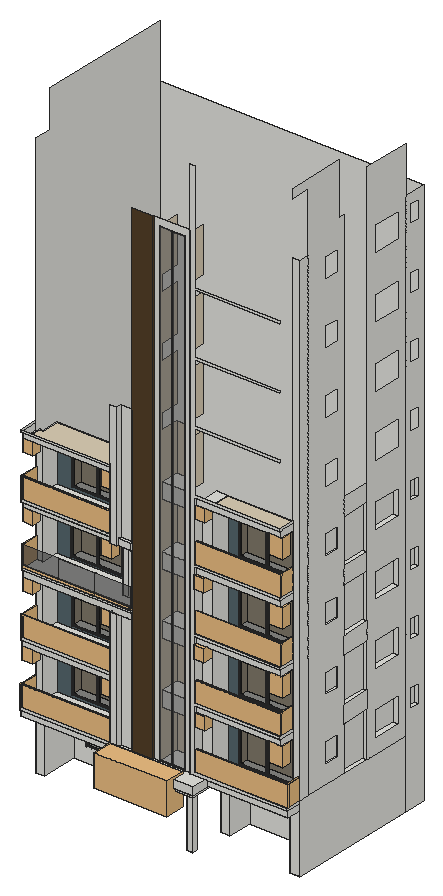
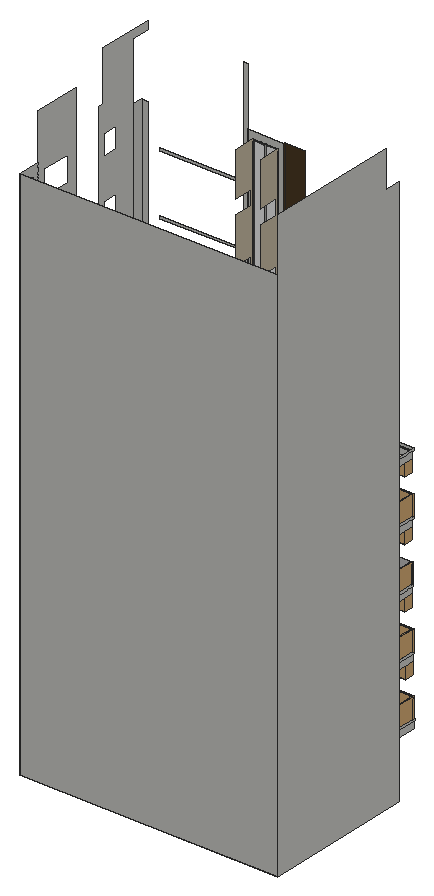
# SketchUp Ruby script. Lengths in inches.
U = 1.inch
M = Sketchup.active_model
def pt(a) = Geom::Point3d.new(a.map { |v| v * U })
def face(e, loops, mat)
  f = e.add_face(loops[0].map { |a| pt(a) })
  loops[1..].each { |l| e.add_face(l.map { |a| pt(a) }).erase! }
  f.material = f.back_material = mat if mat
  f
end
# faces: each face lists its corners as indices into pts; further lists are holes
def faces(e, pts, list, mat = nil) = list.each { |f| face(e, (f[0].is_a?(Array) ? f : [f]).map { |l| l.map { |i| pts[i] } }, mat) }
# xy, xz, yz: faces in a plane at the given z, y or x. An outline is a flat list of corners, or four numbers for a rectangle; further outlines are holes
def ring(l) = l.size == 4 ? [[l[0], l[1]], [l[2], l[1]], [l[2], l[3]], [l[0], l[3]]] : l.each_slice(2).to_a
def flat(e, list, mat, &to3) = list.each { |f| face(e, (f[0].is_a?(Array) ? f : [f]).map { |l| ring(l).map { |u, v| to3.(u, v) } }, mat) }
def xy(e, z, list, mat = nil) = flat(e, list, mat) { |x, y| [x, y, z] }
def xz(e, y, list, mat = nil) = flat(e, list, mat) { |x, z| [x, y, z] }
def yz(e, x, list, mat = nil) = flat(e, list, mat) { |y, z| [x, y, z] }
def lines(e, pts, list) = list.each { |a, b| e.add_line(pt(pts[a]), pt(pts[b])) }
# prism: a flat outline (further loops are holes) pulled along v
def prism(e, loops, v, mat = nil)
  f = face(e, loops, mat); d = Geom::Vector3d.new(v.map { |x| x * U })
  f.pushpull(f.normal.samedirection?(d) ? d.length : -d.length)
end
def box(e, o, s, mat = nil) = prism(e, [[o, [o[0] + s[0], o[1], o[2]], [o[0] + s[0], o[1] + s[1], o[2]], [o[0], o[1] + s[1], o[2]]]], [0, 0, s[2]], mat)
def at(x, y, z, deg = 0) = Geom::Transformation.translation(pt([x, y, z])) * Geom::Transformation.rotation(ORIGIN, Z_AXIS, deg.degrees)
def axes(o, x, y, z) = Geom::Transformation.new([*x, 0, *y, 0, *z, 0, *pt(o).to_a, 1])
def part(name) = M.definitions.add(name)
# library, detail: a bought-in or finely detailed component or shape, given as its bounding box
def library(name, o, s) = part(name).tap { |d| box(d.entities, o, s) }
def detail(e, o, s) = box(e.add_group.entities, o, s)
def put(e, d, t, mat = nil) = e.add_instance(d, t).tap { |i| i.material = mat if mat }
def group(e, t, mat = nil) = e.add_group.tap { |g| g.transformation = t; g.material = mat if mat }.entities
root = M.entities
M.materials.add("Glass_Tinted_Gray").color = [0, 0, 0]
M.materials["Glass_Tinted_Gray"].alpha = 0.125
M.materials.add("Wall Paint Bumpy 01 Blue 100cm").color = [86, 103, 109]
M.materials.add("Wood Planks Pecan 33-81 150cm").color = [83, 63, 40]
M.materials.add("[0135_DarkGray]").color = [81, 81, 81]
M.materials.add("[Mirror 02]").color = [96, 96, 96]
M.materials["[Mirror 02]"].alpha = 0.27
M.materials.add("[Terrazzo Light Blue]").color = [196, 214, 227]
M.materials.add("[Translucent_Glass_Blue]").color = [63, 63, 63]
M.materials["[Translucent_Glass_Blue]"].alpha = 0.35
M.materials.add("metal railing").color = [165, 165, 165]
M.materials.add("plastic2").color = [86, 86, 86]
M.materials.add("warmk").color = [218, 205, 180]
c1 = part("PENTEK_RP Fineline 50S_Sliding_DoorCase_E1")
box(c1.entities,[0,0,0],[1.51,3.66,99.27],"[0135_DarkGray]")
c2 = part("PENTEK_RP Fineline 50S_SlidingDooe_Case_E2")
box(c2.entities,[0,0,0],[96.25,3.66,1.51],"[0135_DarkGray]")
c3 = part("pentek_RP Fineline 50S_SlidingDoor_Case")
put(c3.entities,c1,at(97.76,0,0))
put(c3.entities,c2,at(1.51,0,0))
put(c3.entities,c1,at(0,0,0))
put(c3.entities,c2,at(1.51,0,97.76))
c4 = part("PENTEK_RP Fineline 50S_SlidingDoor_GlazingBead_2")
box(c4.entities,[0,0,0],[0.56,0.59,94.39],"[0135_DarkGray]")
c5 = part("PENTEK_RP Fineline 50S_SlidingDoor_GlazingBead")
box(c5.entities,[0,0,0],[45.47,0.59,0.56],"[0135_DarkGray]")
c6 = part("PENTEK_RP Fineline 50S_SlidingDoor_Glass")
box(c6.entities,[0,0,0],[46.58,0.16,94.39],"Glass_Tinted_Gray")
c7 = part("PENTEK_RP Fineline 50S_SlidingDoor_Leaf_E1")
xy(c7.entities,0,[[0,0,0.93,1.97],[0.93,1.57,1.49,1.97]],"[0135_DarkGray]")
xy(c7.entities,96.25,[[0,0,0.93,0,0.93,1.57,1.49,1.57,1.49,1.97,0,1.97]],"[0135_DarkGray]")
xz(c7.entities,0,[[0,0,0.93,96.25]],"[0135_DarkGray]")
xz(c7.entities,1.57,[[0.93,0,1.49,95.32],[0.93,95.32,1.49,96.25]],"[0135_DarkGray]")
xz(c7.entities,1.97,[[0,0,1.49,96.25]],"[0135_DarkGray]")
yz(c7.entities,0,[[0,0,1.97,96.25]],"[0135_DarkGray]")
yz(c7.entities,0.93,[[0,0,1.57,0.93],[0,0.93,1.57,95.32],[0,95.32,1.57,96.25]],"[0135_DarkGray]")
yz(c7.entities,1.49,[[1.57,0,1.97,95.32],[1.57,95.32,1.97,96.25]],"[0135_DarkGray]")
c8 = part("PENTEK_RP Fineline 50S_SlidingDoor_Leaf_E2")
xy(c8.entities,0,[[0,0,0,1.57,0.56,1.57,0.56,1.97,46.02,1.97,46.02,1.57,46.58,1.57,46.58,0]],"[0135_DarkGray]")
xy(c8.entities,0.93,[[0,0,46.58,1.57]],"[0135_DarkGray]")
xy(c8.entities,1.49,[[0.56,1.57,46.02,1.97]],"[0135_DarkGray]")
xz(c8.entities,0,[[0,0,46.58,0.93]],"[0135_DarkGray]")
xz(c8.entities,1.57,[[0,0,0.56,0.93],[46.02,0,46.58,0.93],[0.56,0.93,46.02,1.49]],"[0135_DarkGray]")
xz(c8.entities,1.97,[[0.56,0,46.02,1.49]],"[0135_DarkGray]")
yz(c8.entities,0,[[0,0,1.57,0.93]],"[0135_DarkGray]")
yz(c8.entities,0.56,[[1.57,0,1.97,0.93],[1.57,0.93,1.97,1.49]],"[0135_DarkGray]")
yz(c8.entities,46.02,[[1.57,0,1.97,0.93],[1.57,0.93,1.97,1.49]],"[0135_DarkGray]")
yz(c8.entities,46.58,[[0,0,1.57,0.93]],"[0135_DarkGray]")
c9 = part("PENTEK_RP Fineline S_SlidingDoor_Leaf1")
put(c9.entities,c4,at(0.93,0,0.93))
put(c9.entities,c4,at(46.96,0,0.93))
put(c9.entities,c5,at(1.49,0,0.93))
put(c9.entities,c6,at(1.49,0.59,0.93),"[Terrazzo Light Blue]")
put(c9.entities,c7,at(0,0,0))
put(c9.entities,c7,axes([48.44,0,0],[-1,0,0],[0,1,0],[0,0,1]))
put(c9.entities,c8,axes([0.93,0,96.25],[1,0,0],[0,1,0],[0,0,-1]))
put(c9.entities,c5,at(1.49,0,94.77))
put(c9.entities,c6,at(1.49,1.42,0.93))
put(c9.entities,c8,at(0.93,0,0))
c10 = part("PENTEK_RP Fineline 50S_SlidingDoor_Leaf2")
put(c10.entities,c6,at(1.49,1.42,0.93))
put(c10.entities,c5,at(1.49,0,94.77))
put(c10.entities,c4,at(46.96,0,0.93))
put(c10.entities,c6,at(1.49,0.59,0.93),"[Mirror 02]")
put(c10.entities,c4,at(0.93,0,0.93))
put(c10.entities,c7,at(0,0,0))
put(c10.entities,c7,axes([48.44,0,0],[-1,0,0],[0,1,0],[0,0,1]))
put(c10.entities,c5,at(1.49,0,0.93))
put(c10.entities,c8,axes([0.93,0,96.25],[1,0,0],[0,1,0],[0,0,-1]))
put(c10.entities,c8,at(0.93,0,0))
c11 = part("PENTEK - Slimmest Steel Sliding Door / Window\#1")
put(c11.entities,c3,at(0,-1.88,-0.09))
put(c11.entities,c9,at(1.51,-2.27,1.42),"[Mirror 02]")
put(c11.entities,c10,at(49.32,-0.3,1.42),"[Mirror 02]")
c12 = library("Group\#2",[0,0,0],[143.94,39.08,63.625])
c13 = library("My+Glass_Railing\#1",[-0.12,0,0],[177.09,2.52,40.9])
c14 = library("My+Glass_Railing\#5",[-0.02,0,0],[34.55,2.52,40.9])
c15 = library("My+Glass_Railing\#4",[-0.125,0,0],[190.28,2.52,40.9])
c16 = library("My+Glass_Railing\#7",[-0.02,0,0],[27.33,2.52,40.9])
c17 = library("Plante \#58",[-0.43,-1.58,0],[20.84,18.06,17.59])
c18 = library("My+Glass_Railing\#6",[-0.02,0,0],[30.48,2.52,40.9])
c19 = library("Railing",[0,0,0],[72,2.52,4.03])
c20 = part("railing plastic")
box(c20.entities,[0,0.75,0],[72,0.26,0.68],"plastic2")
box(c20.entities,[0,0,0],[72,0.26,0.68],"plastic2")
c21 = part("Glass Railing pro\#3")
put(c21.entities,c19,axes([0,0,0],[3.01682,0,0],[0,1,0],[0,0,1]))
put(c21.entities,c20,axes([0,0.75,3.47],[3.01682,0,0],[0,1,0],[0,0,1]))
c22 = part("sheet glass")
box(c22.entities,[0,0,0],[39.37,0.39,39.37],"[Translucent_Glass_Blue]")
c23 = part("glass stretch")
box(c23.entities,[0,0,0],[39.37,0.39,43.31],"[Translucent_Glass_Blue]")
c24 = part("glass frame\#3")
put(c24.entities,c22,axes([0,0,0],[1.8288,0,0],[0,1.016,0],[0,0,1]))
put(c24.entities,c23,axes([216.6,0,0],[0.01552,0,0],[0,1.016,0],[0,0,0.90909]))
put(c24.entities,c22,axes([72.2,0,0],[1.8288,0,0],[0,1.016,0],[0,0,1]))
put(c24.entities,c22,axes([144.4,0,0],[1.8288,0,0],[0,1.016,0],[0,0,1]))
c25 = part("Glass Railing +\#3")
put(c25.entities,c21,at(0,0,0),"metal railing")
put(c25.entities,c24,at(0,1.0625,1.53),"metal railing")
c26 = part("My+Glass_Railing\#3")
put(c26.entities,c25,at(-0.14,0,0))
xy(root,0,[[334.13,20.33,347.71,30.2],[0,64.57,0,372.25,524.5,372.25,524.5,64.57,504.24,64.57,504.24,145.15,360.33,145.15,360.33,96.59,341.3125,96.59,341.3125,182.74,296.85,182.74,296.85,238.43,218.16,238.43,218.16,182.74,178.39,182.74,178.39,137.57,16.9,137.57,16.9,64.57]])
xy(root,29.84,[[40.75,137.57,164.84,174.7]])
xy(root,46.24,[[388.1875,145.15,476.86,151.81]])
xy(root,85.5,[[218.16,182.74,296.85,238.43]])
xy(root,100.83,[[16.9,114.72,16.9,137.57,40.75,137.57,40.75,174.7,164.84,174.7,164.84,137.57,178.39,137.57,178.39,114.72],[360.33,114.72,360.33,145.15,388.1875,145.15,388.1875,151.81,476.86,151.81,476.86,145.15,504.24,145.15,504.24,114.72]])
xy(root,108.375,[[[178.39,4.65,178.39,182.74,341.3125,182.74,341.3125,96.59,358.96,96.59,358.96,4.65],[334.13,20.33,347.71,30.2]]])
xy(root,115.74,[[178.39,0,178.39,4.65,358.96,4.65,358.96,96.59,362.95,96.59,362.95,0]])
xy(root,117.87,[[0,27.71,0,64.57,16.9,64.57,16.9,114.72,178.39,114.72,178.39,27.71]])
xy(root,117.87,[[362.95,34.48,362.95,96.59,360.33,96.59,360.33,114.72,504.24,114.72,504.24,64.57,524.5,64.57,524.5,34.48]],"warmk")
xy(root,130.08,[[178.39,0,362.95,0,362.95,32.16,332.22,32.16,332.22,34.48,258.12,34.48,258.12,32.07,217.21,32.07,217.21,36.36,190.43,36.36,190.43,27.71,178.39,27.71],[0,24.45,176.99,27.71],[332.22,32.16,340.89,34.48],[362.95,32.16,524.5,34.48],[269.54,34.48,320.5,78.02]])
xy(root,134.96,[[0,24.45,176.99,24.45,176.99,99,14.45,99,14.45,64.57,0,64.57],[340.89,32.16,524.5,32.16,524.5,63.53,511.32,63.53,511.32,87.39,362.73,87.39,362.73,49.47,340.89,49.47],[515.49,172.42,524.5,231.18]])
xy(root,139.15,[[384.04,87.39,497.86,108.38],[43.39,99,146.83,121.27]])
xy(root,163.08,[[512.56,251.74,524.5,310.65]])
xy(root,171.34,[[518.78,127.53,524.5,159.82]])
xy(root,177.77,[[516.25,338.3,524.5,358.82]])
xy(root,211.92,[[518.78,127.53,524.5,159.82]])
xy(root,214.26,[[512.56,251.74,524.5,310.65]])
xy(root,214.8,[[516.25,338.3,524.5,358.82]])
xy(root,222.93,[[269.54,39.85,320.5,78.02],[384.04,87.39,497.86,108.38],[43.39,99,146.83,121.27]],"warmk")
xy(root,224.94,[[515.49,172.42,524.5,231.18]])
xy(root,241.17,[[0,29.32,0,64.57,7.22,64.57,7.22,35.38,176.99,35.38,176.99,29.32],[340.89,49.47,362.73,87.39]])
xy(root,241.17,[[340.89,34.48,340.89,49.47,362.73,49.47,362.73,87.39,511.32,87.39,511.32,34.48]],"warmk")
xy(root,244.6,[[7.22,35.38,7.22,64.57,14.45,64.57,14.45,99,176.99,99,176.99,35.38]],"warmk")
xy(root,253.38,[[0,26.39,176.99,29.32],[340.89,32.16,511.32,34.48],[269.54,39.85,320.5,78.02]])
xy(root,258.26,[[0,26.39,176.99,26.39,176.99,99,14.45,99,14.45,64.57,0,64.57],[340.89,32.16,511.32,32.16,511.32,87.39,362.73,87.39,362.73,49.47,340.89,49.47],[515.49,172.42,524.5,231.18]])
xy(root,262.45,[[384.04,87.39,497.86,108.38],[43.39,99,146.83,121.27]])
xy(root,286.38,[[512.56,251.74,524.5,310.65]])
xy(root,294.64,[[518.78,127.53,524.5,159.82]])
xy(root,301.0625,[[516.25,338.3,524.5,358.82]])
xy(root,335.22,[[518.78,127.53,524.5,159.82]])
xy(root,337.5625,[[512.56,251.74,524.5,310.65]])
xy(root,338.1,[[516.25,338.3,524.5,358.82]])
xy(root,346.23,[[269.54,39.85,320.5,78.02],[384.04,87.39,497.86,108.38],[43.39,99,146.83,121.27]],"warmk")
xy(root,346.5625,[[515.49,172.42,524.5,231.18]])
xy(root,364.47,[[176.99,27.71,190.43,30.65],[0,30.65,0,64.57,7.22,64.57,7.22,35.38,176.99,35.38,176.99,30.65],[190.43,30.65,217.21,36.36],[340.89,49.47,362.73,87.39]])
xy(root,364.47,[[340.89,34.48,340.89,49.47,362.73,49.47,362.73,87.39,511.32,87.39,511.32,34.48]],"warmk")
xy(root,367.9,[[7.22,35.38,7.22,64.57,14.45,64.57,14.45,99,176.99,99,176.99,35.38]],"warmk")
xy(root,376.68,[[0,28.33,217.21,30.65],[340.89,32.16,511.32,34.48],[269.54,39.85,320.5,78.02]])
xy(root,381.56,[[0,28.33,217.21,28.33,217.21,58.85,176.99,58.85,176.99,99,14.45,99,14.45,64.57,0,64.57],[340.89,32.16,511.32,32.16,511.32,87.39,362.73,87.39,362.73,49.47,340.89,49.47],[515.49,172.42,524.5,231.18]])
xy(root,385.74,[[384.04,87.39,497.86,108.38],[43.39,99,146.83,121.27]])
xy(root,409.68,[[512.56,251.74,524.5,310.65]])
xy(root,417.94,[[518.78,127.53,524.5,159.82]])
xy(root,424.36,[[516.25,338.3,524.5,358.82]])
xy(root,458.51,[[518.78,127.53,524.5,159.82]])
xy(root,460.86,[[512.56,251.74,524.5,310.65]])
xy(root,461.4,[[516.25,338.3,524.5,358.82]])
xy(root,469.53,[[269.54,39.85,320.5,78.02],[384.04,87.39,497.86,108.38],[43.39,99,146.83,121.27]],"warmk")
xy(root,471.54,[[515.49,172.42,524.5,231.18]])
xy(root,487.77,[[176.99,27.71,176.99,58.85,217.21,58.85,217.21,29.59,190.43,29.59,190.43,27.71],[0,30.65,0,64.57,7.22,64.57,7.22,35.38,176.99,35.38,176.99,30.65],[340.89,49.47,362.73,87.39]])
xy(root,487.77,[[340.89,34.48,340.89,49.47,362.73,49.47,362.73,87.39,511.32,87.39,511.32,34.48]],"warmk")
xy(root,491.19,[[7.22,35.38,7.22,64.57,14.45,64.57,14.45,99,176.99,99,176.99,35.38]],"warmk")
xy(root,499.97,[[0,26.52,176.99,30.65],[190.43,29.59,217.21,36.36],[340.89,32.16,511.32,34.48],[269.54,39.85,320.5,78.02]])
xy(root,504.86,[[0,26.52,176.99,26.52,176.99,99,14.45,99,14.45,64.57,0,64.57],[340.89,32.16,511.32,32.16,511.32,87.39,362.73,87.39,362.73,49.47,340.89,49.47],[515.49,172.42,524.5,231.18]])
xy(root,509.04,[[384.04,87.39,497.86,108.38],[43.39,99,146.83,121.27]])
xy(root,532.98,[[512.56,251.74,524.5,310.65]])
xy(root,541.24,[[518.78,127.53,524.5,159.82]])
xy(root,547.66,[[516.25,338.3,524.5,358.82]])
xy(root,581.8125,[[518.78,127.53,524.5,159.82]])
xy(root,584.16,[[512.56,251.74,524.5,310.65]])
xy(root,584.69,[[516.25,338.3,524.5,358.82]])
xy(root,592.83,[[269.54,39.85,320.5,78.02],[384.04,87.39,497.86,108.38],[43.39,99,146.83,121.27]],"warmk")
xy(root,593.16,[[515.49,172.42,524.5,231.18]])
xy(root,611.0625,[[0,30.65,0,64.57,7.22,64.57,7.22,35.38,176.99,35.38,176.99,30.65],[340.89,49.47,362.73,87.39]])
xy(root,611.0625,[[340.89,34.48,340.89,49.47,362.73,49.47,362.73,87.39,511.32,87.39,511.32,34.48]],"warmk")
xy(root,614.49,[[7.22,35.38,7.22,64.57,14.45,64.57,14.45,99,176.99,99,176.99,35.38]],"warmk")
xy(root,623.27,[[0,26.52,176.99,30.65],[340.89,32.16,511.32,34.48],[269.54,39.85,320.5,78.02]])
xz(root,0,[[178.39,115.74,362.95,130.08]])
xz(root,4.65,[[178.39,108.375,358.96,115.74]])
xz(root,20.33,[[334.13,0,347.71,108.375]])
xz(root,24.45,[[0,130.08,176.99,134.96]])
xz(root,26.39,[[0,253.38,176.99,258.26]])
xz(root,26.52,[[0,499.97,176.99,504.86],[0,623.27,176.99,628.16]])
xz(root,27.71,[[0,117.87,176.99,130.08],[176.99,117.87,178.39,117.87,178.39,130.08,190.43,130.08,190.43,364.47,176.99,364.47],[176.99,487.77,190.43,734.36]])
xz(root,28.33,[[0,376.68,217.21,381.56]])
xz(root,29.32,[[0,241.17,176.99,253.38]])
xz(root,29.59,[[190.43,487.77,217.21,499.97]])
xz(root,30.2,[[334.13,0,347.71,108.375]])
xz(root,30.65,[[0,364.47,217.21,376.68],[0,487.77,176.99,499.97],[0,611.0625,176.99,623.27]])
xz(root,32.07,[[217.21,130.08,258.12,1096.46]],"Wood Planks Pecan 33-81 150cm")
xz(root,32.16,[[332.22,130.08,524.5,130.08,524.5,134.96,340.89,134.96,340.89,253.38,511.32,253.38,511.32,258.26,340.89,258.26,340.89,376.68,511.32,376.68,511.32,381.56,340.89,381.56,340.89,499.97,511.32,499.97,511.32,504.86,340.89,504.86,340.89,623.27,511.32,623.27,511.32,628.16,340.89,628.16,340.89,746.57,511.32,746.57,511.32,751.45,340.89,751.45,340.89,869.87,511.32,869.87,511.32,874.75,340.89,874.75,340.89,993.17,511.32,993.17,511.32,998.05,340.89,998.05,340.89,1215.07,332.22,1215.07]])
xz(root,34.48,[[362.95,117.87,524.5,130.08],[258.12,130.08,269.54,130.08,269.54,1082.38,320.5,1082.38,320.5,130.08,332.22,130.08,332.22,1096.46,258.12,1096.46],[340.89,241.17,511.32,253.38],[340.89,364.47,511.32,376.68],[340.89,487.77,511.32,499.97],
  [340.89,611.0625,511.32,623.27]])
xz(root,35.38,[[7.22,241.17,176.99,244.6],[7.22,364.47,176.99,367.9],[7.22,487.77,176.99,491.19],[7.22,611.0625,176.99,614.49]])
xz(root,36.36,[[190.43,130.08,217.21,364.47],[190.43,499.97,217.21,734.36]])
xz(root,39.85,[[269.54,222.93,320.5,253.38],[269.54,346.23,320.5,376.68],[269.54,469.53,320.5,499.97],[269.54,592.83,320.5,623.27]])
xz(root,49.47,[[340.89,134.96,362.73,241.17],[340.89,258.26,362.73,364.47],[340.89,381.56,362.73,487.77],[340.89,504.86,362.73,611.0625]])
xz(root,58.85,[[176.99,381.56,187.04,487.77],[187.04,381.56,217.21,487.77]])
xz(root,63.53,[[511.32,134.96,524.5,1096.46]])
xz(root,64.57,[[0,0,16.9,117.87],[504.24,0,524.5,117.87],[0,134.96,14.45,134.96,14.45,244.6,7.22,244.6,7.22,241.17,0,241.17],[0,258.26,14.45,258.26,14.45,367.9,7.22,367.9,7.22,364.47,0,364.47],[0,381.56,14.45,381.56,14.45,491.19,7.22,491.19,7.22,487.77,0,487.77],
  [0,504.86,14.45,504.86,14.45,614.49,7.22,614.49,7.22,611.0625,0,611.0625]])
xz(root,78.02,[[269.54,130.08,320.5,222.93],[269.54,253.38,320.5,346.23],[269.54,376.68,320.5,469.53],[269.54,499.97,320.5,592.83],[269.54,623.27,320.5,716.125]],"warmk")
xz(root,87.39,[[[362.73,134.96,511.32,241.17],[384.04,139.15,497.86,222.93]],[[362.73,258.26,511.32,364.47],[384.04,262.45,497.86,346.23]],[[362.73,381.56,511.32,487.77],[384.04,385.74,497.86,469.53]],[[362.73,504.86,511.32,611.0625],[384.04,509.04,497.86,592.83]]],"Wall Paint Bumpy 01 Blue 100cm")
xz(root,96.59,[[341.3125,0,360.33,108.375],[358.96,108.375,360.33,115.74],[360.33,115.74,362.95,117.87]])
xz(root,99,[[[14.45,134.96,176.99,244.6],[43.39,139.15,146.83,222.93]],[[14.45,258.26,176.99,367.9],[43.39,262.45,146.83,346.23]],[[14.45,381.56,176.99,491.19],[43.39,385.74,146.83,469.53]],[[14.45,504.86,176.99,614.49],[43.39,509.04,146.83,592.83]]],"Wall Paint Bumpy 01 Blue 100cm")
xz(root,108.38,[[384.04,139.15,497.86,222.93],[384.04,262.45,497.86,346.23],[384.04,385.74,497.86,469.53],[384.04,509.04,497.86,592.83]],"warmk")
xz(root,114.72,[[16.9,100.83,178.39,117.87],[360.33,100.83,504.24,117.87]])
xz(root,121.27,[[43.39,139.15,146.83,222.93],[43.39,262.45,146.83,346.23],[43.39,385.74,146.83,469.53],[43.39,509.04,146.83,592.83]],"warmk")
xz(root,127.53,[[518.78,171.34,524.5,211.92],[518.78,294.64,524.5,335.22],[518.78,417.94,524.5,458.51],[518.78,541.24,524.5,581.8125]])
xz(root,137.57,[[16.9,0,178.39,0,178.39,100.83,164.84,100.83,164.84,29.84,40.75,29.84,40.75,100.83,16.9,100.83]])
xz(root,145.15,[[360.33,0,504.24,0,504.24,100.83,476.86,100.83,476.86,46.24,388.1875,46.24,388.1875,100.83,360.33,100.83]])
xz(root,151.81,[[388.1875,46.24,476.86,100.83]])
xz(root,159.82,[[518.78,171.34,524.5,211.92],[518.78,294.64,524.5,335.22],[518.78,417.94,524.5,458.51],[518.78,541.24,524.5,581.8125]])
xz(root,172.42,[[515.49,134.96,524.5,224.94],[515.49,258.26,524.5,346.5625],[515.49,381.56,524.5,471.54],[515.49,504.86,524.5,593.16]])
xz(root,174.7,[[40.75,29.84,164.84,100.83]])
xz(root,182.74,[[178.39,0,218.16,0,218.16,85.5,296.85,85.5,296.85,0,341.3125,0,341.3125,108.375,178.39,108.375]])
xz(root,231.18,[[515.49,134.96,524.5,224.94],[515.49,258.26,524.5,346.5625],[515.49,381.56,524.5,471.54],[515.49,504.86,524.5,593.16]])
xz(root,238.43,[[218.16,0,296.85,85.5]])
xz(root,251.74,[[512.56,163.08,524.5,214.26],[512.56,286.38,524.5,337.5625],[512.56,409.68,524.5,460.86],[512.56,532.98,524.5,584.16]])
xz(root,310.65,[[512.56,163.08,524.5,214.26],[512.56,286.38,524.5,337.5625],[512.56,409.68,524.5,460.86],[512.56,532.98,524.5,584.16]])
xz(root,338.3,[[516.25,177.77,524.5,214.8],[516.25,301.0625,524.5,338.1],[516.25,424.36,524.5,461.4],[516.25,547.66,524.5,584.69]])
xz(root,358.82,[[516.25,177.77,524.5,214.8],[516.25,301.0625,524.5,338.1],[516.25,424.36,524.5,461.4],[516.25,547.66,524.5,584.69]])
xz(root,372.25,[[0,0,524.5,1096.46]])
yz(root,0,[[64.57,0,64.57,1130.13,99,1130.13,99,1204.84,372.25,1204.84,372.25,0],[27.71,117.87,64.57,130.08],[24.45,130.08,64.57,134.96],[29.32,241.17,64.57,253.38],[26.39,253.38,64.57,258.26],
  [30.65,364.47,64.57,376.68],[28.33,376.68,64.57,381.56],[30.65,487.77,64.57,499.97],[26.52,499.97,64.57,504.86],[30.65,611.0625,64.57,623.27],
  [26.52,623.27,64.57,628.16]])
yz(root,7.22,[[35.38,241.17,64.57,244.6],[35.38,364.47,64.57,367.9],[35.38,487.77,64.57,491.19],[35.38,611.0625,64.57,614.49]])
yz(root,14.45,[[64.57,134.96,99,244.6],[64.57,258.26,99,367.9],[64.57,381.56,99,491.19],[64.57,504.86,99,614.49]])
yz(root,16.9,[[64.57,0,137.57,0,137.57,100.83,114.72,100.83,114.72,117.87,64.57,117.87]])
yz(root,40.75,[[137.57,29.84,174.7,100.83]])
yz(root,43.39,[[99,139.15,121.27,222.93],[99,262.45,121.27,346.23],[99,385.74,121.27,469.53],[99,509.04,121.27,592.83]],"warmk")
yz(root,146.83,[[99,139.15,121.27,222.93],[99,262.45,121.27,346.23],[99,385.74,121.27,469.53],[99,509.04,121.27,592.83]],"warmk")
yz(root,164.84,[[137.57,29.84,174.7,100.83]])
yz(root,176.99,[[24.45,130.08,27.71,134.96],[27.71,241.17,29.32,253.38],[26.39,253.38,27.71,258.26],[27.71,487.77,30.65,499.97],[35.38,487.77,58.85,491.19],
  [26.52,499.97,27.71,504.86],[27.71,611.0625,30.65,623.27],[26.52,623.27,27.71,628.16]])
yz(root,176.99,[[27.71,134.96,27.71,241.17,35.38,241.17,35.38,244.6,99,244.6,99,134.96],[27.71,258.26,27.71,364.47,35.38,364.47,35.38,367.9,99,367.9,99,258.26],[58.85,381.56,99,491.19],[27.71,504.86,27.71,611.0625,35.38,611.0625,35.38,614.49,99,614.49,99,504.86]],"Wall Paint Bumpy 01 Blue 100cm")
yz(root,178.39,[[137.57,0,182.74,108.375],[114.72,100.83,137.57,108.375],[4.65,108.375,4.65,115.74,0,115.74,0,130.08,27.71,130.08,27.71,117.87,114.72,117.87,114.72,108.375]])
yz(root,190.43,[[27.71,130.08,36.36,364.47],[27.71,487.77,29.59,487.77,29.59,499.97,36.36,499.97,36.36,734.36,27.71,734.36]])
yz(root,217.21,[[32.07,130.08,36.36,364.47],[30.65,364.47,32.07,376.68],[28.33,376.68,32.07,381.56],[32.07,381.56,58.85,487.77],[29.59,487.77,32.07,499.97],
  [32.07,499.97,36.36,734.36]])
yz(root,218.16,[[182.74,0,238.43,85.5]])
yz(root,258.12,[[32.07,130.08,34.48,1096.46]],"Wood Planks Pecan 33-81 150cm")
yz(root,269.54,[[34.48,130.08,78.02,130.08,78.02,222.93,39.85,222.93,39.85,253.38,78.02,253.38,78.02,346.23,39.85,346.23,39.85,376.68,78.02,376.68,78.02,469.53,39.85,469.53,39.85,499.97,78.02,499.97,78.02,592.83,39.85,592.83,39.85,623.27,78.02,623.27,78.02,716.125,39.85,716.125,39.85,746.57,78.02,746.57,78.02,839.42,39.85,839.42,39.85,869.87,78.02,869.87,78.02,962.72,39.85,962.72,39.85,993.17,78.02,993.17,78.02,1082.38,34.48,1082.38]],"warmk")
yz(root,296.85,[[182.74,0,238.43,85.5]])
yz(root,320.5,[[34.48,130.08,34.48,1082.38,78.02,1082.38,78.02,993.17,39.85,993.17,39.85,962.72,78.02,962.72,78.02,869.87,39.85,869.87,39.85,839.42,78.02,839.42,78.02,746.57,39.85,746.57,39.85,716.125,78.02,716.125,78.02,623.27,39.85,623.27,39.85,592.83,78.02,592.83,78.02,499.97,39.85,499.97,39.85,469.53,78.02,469.53,78.02,376.68,39.85,376.68,39.85,346.23,78.02,346.23,78.02,253.38,39.85,253.38,39.85,222.93,78.02,222.93,78.02,130.08]],"warmk")
yz(root,332.22,[[32.16,130.08,34.48,1096.46]])
yz(root,334.13,[[20.33,0,30.2,108.375]])
yz(root,340.89,[[32.16,134.96,49.47,134.96,49.47,241.17,34.48,241.17,34.48,253.38,32.16,253.38],[32.16,258.26,49.47,258.26,49.47,364.47,34.48,364.47,34.48,376.68,32.16,376.68],[32.16,381.56,49.47,381.56,49.47,487.77,34.48,487.77,34.48,499.97,32.16,499.97],[32.16,504.86,49.47,504.86,49.47,611.0625,34.48,611.0625,34.48,623.27,32.16,623.27]])
yz(root,341.3125,[[96.59,0,182.74,108.375]])
yz(root,347.71,[[20.33,0,30.2,108.375]])
yz(root,358.96,[[4.65,108.375,96.59,115.74]])
yz(root,360.33,[[96.59,0,145.15,0,145.15,100.83,114.72,100.83,114.72,108.375,96.59,108.375],[96.59,108.375,114.72,117.87]])
yz(root,362.73,[[49.47,134.96,87.39,241.17],[49.47,258.26,87.39,364.47],[49.47,381.56,87.39,487.77],[49.47,504.86,87.39,611.0625]])
yz(root,362.95,[[0,115.74,96.59,115.74,96.59,117.87,34.48,117.87,34.48,130.08,0,130.08]])
yz(root,384.04,[[87.39,139.15,108.38,222.93],[87.39,262.45,108.38,346.23],[87.39,385.74,108.38,469.53],[87.39,509.04,108.38,592.83]],"warmk")
yz(root,388.1875,[[145.15,46.24,151.81,100.83]])
yz(root,476.86,[[145.15,46.24,151.81,100.83]])
yz(root,497.86,[[87.39,139.15,108.38,222.93],[87.39,262.45,108.38,346.23],[87.39,385.74,108.38,469.53],[87.39,509.04,108.38,592.83]],"warmk")
yz(root,504.24,[[64.57,0,64.57,117.87,114.72,117.87,114.72,100.83,145.15,100.83,145.15,0]])
yz(root,511.32,[[63.53,134.96,87.39,241.17],[34.48,241.17,63.53,253.38],[32.16,253.38,63.53,258.26],[63.53,258.26,87.39,364.47],[34.48,364.47,63.53,376.68],
  [32.16,376.68,63.53,381.56],[63.53,381.56,87.39,487.77],[34.48,487.77,63.53,499.97],[32.16,499.97,63.53,504.86],[63.53,504.86,87.39,611.0625],
  [34.48,611.0625,63.53,623.27],[32.16,623.27,63.53,628.16]])
yz(root,512.56,[[251.74,163.08,310.65,214.26],[251.74,286.38,310.65,337.5625],[251.74,409.68,310.65,460.86],[251.74,532.98,310.65,584.16]])
yz(root,515.49,[[172.42,134.96,231.18,224.94],[172.42,258.26,231.18,346.5625],[172.42,381.56,231.18,471.54],[172.42,504.86,231.18,593.16]])
yz(root,516.25,[[338.3,177.77,358.82,214.8],[338.3,301.0625,358.82,338.1],[338.3,424.36,358.82,461.4],[338.3,547.66,358.82,584.69]])
yz(root,518.78,[[127.53,171.34,159.82,211.92],[127.53,294.64,159.82,335.22],[127.53,417.94,159.82,458.51],[127.53,541.24,159.82,581.8125]])
yz(root,524.5,[[64.57,0,326.45,0,326.45,134.96,63.53,134.96,63.53,117.87,64.57,117.87],[[326.45,0,372.25,1096.46],[338.3,794.25,358.82,831.29],[338.3,670.96,358.82,707.99],[338.3,917.55,358.82,954.59],[338.3,1040.85,358.82,1077.89],[338.3,177.77,358.82,214.8],[338.3,424.36,358.82,461.4],[338.3,301.0625,358.82,338.1],[338.3,547.66,358.82,584.69]],[34.48,117.87,63.53,130.08],[32.16,130.08,63.53,134.96],[[84.62,134.96,172.42,134.96,172.42,1130.13,161.36,1130.13,161.36,1232.51,46.41,1232.51,46.41,1215.07,84.62,1215.07],[127.53,664.54,159.82,705.11],[127.53,787.83,159.82,828.41],[127.53,417.94,159.82,458.51],[127.53,171.34,159.82,211.92],[127.53,911.13,159.82,951.7],[127.53,294.64,159.82,335.22],[127.53,541.24,159.82,581.8125],[127.53,1034.43,159.82,1075]],
  [63.53,134.96,84.62,1096.46],[[231.18,134.96,326.45,1189.91],[251.74,779.57,310.65,830.75],[251.74,409.68,310.65,460.86],[251.74,1026.17,310.65,1077.35],[251.74,163.08,310.65,214.26],[251.74,656.28,310.65,707.45],[251.74,286.38,310.65,337.5625],[251.74,902.87,310.65,954.05],[251.74,532.98,310.65,584.16]],[172.42,224.94,231.18,258.26],[172.42,346.5625,231.18,381.56],[172.42,471.54,231.18,504.86],
  [172.42,593.16,231.18,628.16]])
put(root,c11,axes([40.75,139.12,29.91],[1.24993,0,0],[0,0.6832,0],[0,0,0.71942]))
put(root,c11,axes([388.3,146.7,46.29],[0.89208,0,0],[0,0.6832,0],[0,0,0.54983]))
put(root,c12,at(179.09,-14.5,70.12))
g1 = group(root,at(269.54,34.48,130.08))
xy(g1,0,[[0,0,25.48,0.92],[25.48,0,50.96,0.92]])
xy(g1,952.3,[[0,0,25.48,0.92],[25.48,0,50.96,0.92]])
xz(g1,0,[[[0,0,25.48,952.3],[1.0625,0.86,24.42,951.44]],[[25.48,0,50.96,952.3],[26.64,0.9375,49.8,951.37]]])
xz(g1,0,[[1.0625,0.86,24.42,951.44],[26.64,0.9375,49.8,951.37]],"[Mirror 02]")
xz(g1,0.92,[[0,0,25.48,952.3],[25.48,0,50.96,952.3]],"[Mirror 02]")
yz(g1,0,[[0,0,0.92,952.3]])
yz(g1,25.48,[[0,0,0.92,952.3]])
yz(g1,50.96,[[0,0,0.92,952.3]])
put(root,c13,at(0.02,25.44,134.96))
put(root,c14,at(2.71,26.93,134.96,90))
put(root,c15,at(334.35,33.63,134.96))
put(root,c16,at(524.5,36.23,134.96,90))
put(root,c11,axes([43.39,100.28,139.23],[1.04197,0,0],[0,0.6832,0],[0,0,0.84587]))
put(root,c11,axes([384.04,88.68,139.23],[1.14656,0,0],[0,0.6832,0],[0,0,0.84587]))
put(root,c17,axes([487.2,36.05,203.71],[1.35,0,0],[0,1,0],[0,0,2.13]))
put(root,c17,axes([156.58,30.9,211.58],[1,0,0],[0,1,0],[0,0,1.6827]))
put(root,c17,axes([341.32,33.73,216.2],[1,0,0],[0,1,0],[0,0,1.42]))
put(root,c17,axes([0.43,30.9,216.2],[1,0,0],[0,1,0],[0,0,1.42]))
put(root,c13,at(0.02,27.38,258.26))
put(root,c13,at(334.34,33.63,258.26))
put(root,c14,at(2.71,28.86,258.26,90))
put(root,c18,at(511.32,36.23,258.26,90))
put(root,c11,axes([43.39,100.28,262.52],[1.04197,0,0],[0,0.6832,0],[0,0,0.84587]))
put(root,c11,axes([384.04,88.68,262.8],[1.14656,0,0],[0,0.6832,0],[0,0,0.84587]))
put(root,c17,axes([487.2,36.05,327.01],[1.35,0,0],[0,1,0],[0,0,2.13]))
put(root,c17,axes([156.58,32.23,334.875],[1,0,0],[0,1,0],[0,0,1.6827]))
put(root,c17,axes([342.32,30.67,339.49],[1,0,0],[0,1,0],[0,0,1.42]))
put(root,c17,axes([0.43,32.23,339.49],[1,0,0],[0,1,0],[0,0,1.42]))
put(root,c13,at(334.34,33.63,381.54))
put(root,c26,at(0.14,29,381.56))
put(root,c14,at(2.7,29.8125,381.56,90))
put(root,c18,at(511.32,36.23,381.56,90))
put(root,c11,axes([43.39,99,385.74],[1.04197,0,0],[0,0.6832,0],[0,0,0.84587]))
put(root,c11,axes([384.04,88.68,386.1],[1.14656,0,0],[0,0.6832,0],[0,0,0.84587]))
put(root,c17,axes([487.2,36.05,450.3],[1.35,0,0],[0,1,0],[0,0,2.13]))
put(root,c17,axes([156.58,32.23,458.17],[1,0,0],[0,1,0],[0,0,1.6827]))
put(root,c17,axes([341.32,31.73,462.15],[1,0,0],[0,1,0],[0,0,1.42]))
put(root,c17,axes([0.43,32.23,462.79],[1,0,0],[0,1,0],[0,0,1.42]))
put(root,c13,at(0.02,27.5,504.86))
put(root,c14,at(2.71,28.99,504.86,90))
put(root,c18,at(511.32,36.23,504.86,90))
put(root,c13,at(334.34,33.63,504.91))
put(root,c11,axes([43.39,100.55,509.12],[1.04197,0,0],[0,0.6832,0],[0,0,0.84587]))
put(root,c11,axes([384.04,88.68,509.4],[1.14656,0,0],[0,0.6832,0],[0,0,0.84587]))
put(root,c17,axes([487.2,36.05,573.6],[1.35,0,0],[0,1,0],[0,0,2.13]))
put(root,c17,axes([156.58,32.23,581.47],[1,0,0],[0,1,0],[0,0,1.6827]))
put(root,c17,axes([341.32,33.73,586.09],[1,0,0],[0,1,0],[0,0,1.42]))
put(root,c17,axes([0.43,32.23,586.09],[1,0,0],[0,1,0],[0,0,1.42]))
